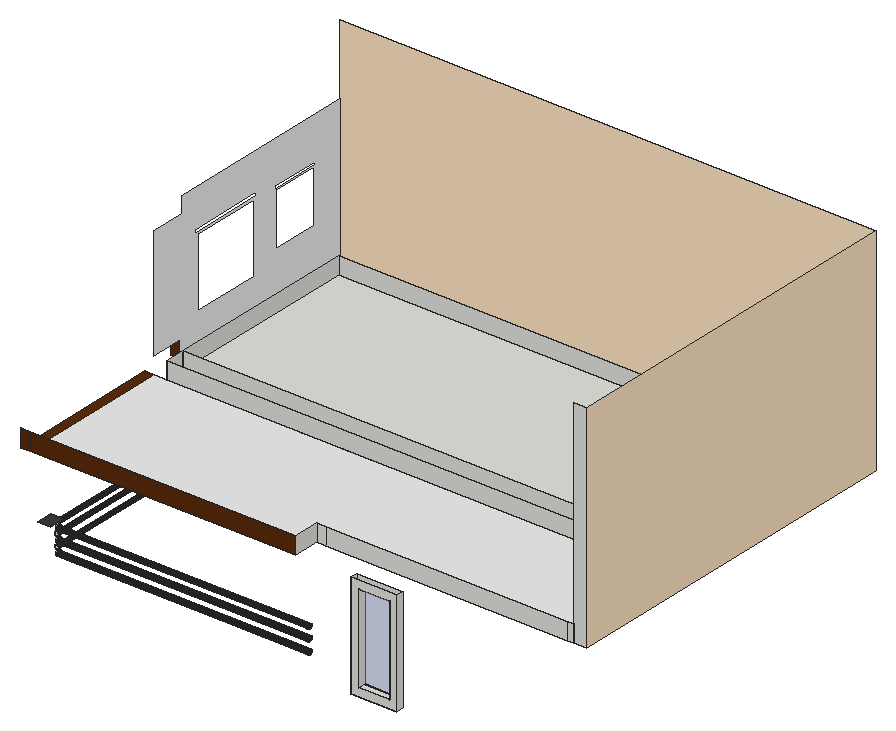
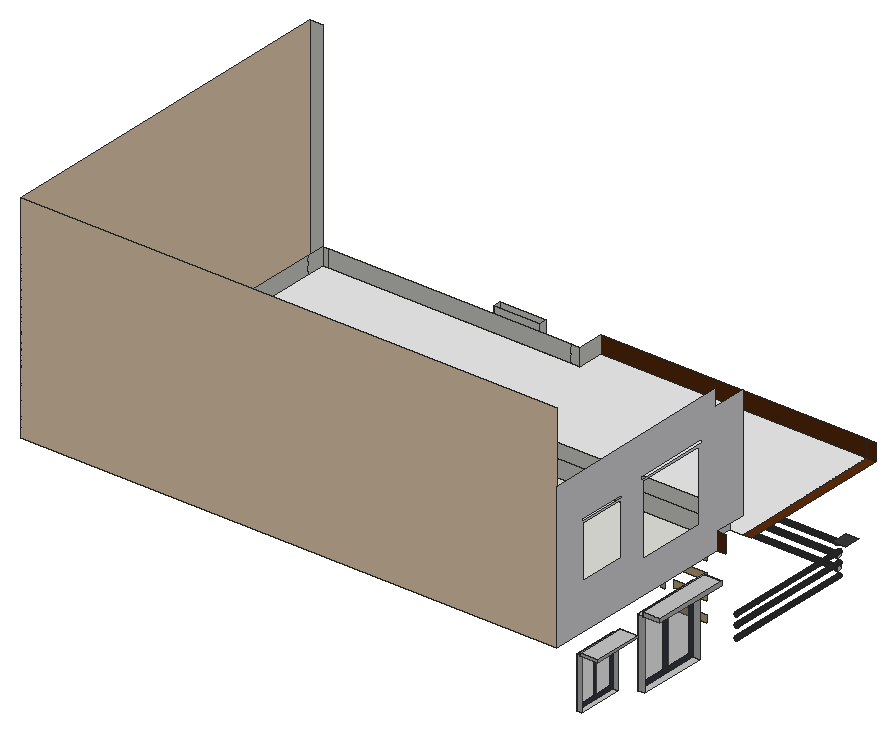
# SketchUp Ruby script. Lengths in inches.
U = 1.inch
M = Sketchup.active_model
def pt(a) = Geom::Point3d.new(a.map { |v| v * U })
def face(e, loops, mat)
  f = e.add_face(loops[0].map { |a| pt(a) })
  loops[1..].each { |l| e.add_face(l.map { |a| pt(a) }).erase! }
  f.material = f.back_material = mat if mat
  f
end
# faces: each face lists its corners as indices into pts; further lists are holes
def faces(e, pts, list, mat = nil) = list.each { |f| face(e, (f[0].is_a?(Array) ? f : [f]).map { |l| l.map { |i| pts[i] } }, mat) }
# xy, xz, yz: faces in a plane at the given z, y or x. An outline is a flat list of corners, or four numbers for a rectangle; further outlines are holes
def ring(l) = l.size == 4 ? [[l[0], l[1]], [l[2], l[1]], [l[2], l[3]], [l[0], l[3]]] : l.each_slice(2).to_a
def flat(e, list, mat, &to3) = list.each { |f| face(e, (f[0].is_a?(Array) ? f : [f]).map { |l| ring(l).map { |u, v| to3.(u, v) } }, mat) }
def xy(e, z, list, mat = nil) = flat(e, list, mat) { |x, y| [x, y, z] }
def xz(e, y, list, mat = nil) = flat(e, list, mat) { |x, z| [x, y, z] }
def yz(e, x, list, mat = nil) = flat(e, list, mat) { |y, z| [x, y, z] }
def lines(e, pts, list) = list.each { |a, b| e.add_line(pt(pts[a]), pt(pts[b])) }
# prism: a flat outline (further loops are holes) pulled along v
def prism(e, loops, v, mat = nil)
  f = face(e, loops, mat); d = Geom::Vector3d.new(v.map { |x| x * U })
  f.pushpull(f.normal.samedirection?(d) ? d.length : -d.length)
end
def box(e, o, s, mat = nil) = prism(e, [[o, [o[0] + s[0], o[1], o[2]], [o[0] + s[0], o[1] + s[1], o[2]], [o[0], o[1] + s[1], o[2]]]], [0, 0, s[2]], mat)
def at(x, y, z, deg = 0) = Geom::Transformation.translation(pt([x, y, z])) * Geom::Transformation.rotation(ORIGIN, Z_AXIS, deg.degrees)
def axes(o, x, y, z) = Geom::Transformation.new([*x, 0, *y, 0, *z, 0, *pt(o).to_a, 1])
def part(name) = M.definitions.add(name)
# library, detail: a bought-in or finely detailed component or shape, given as its bounding box
def library(name, o, s) = part(name).tap { |d| box(d.entities, o, s) }
def detail(e, o, s) = box(e.add_group.entities, o, s)
def put(e, d, t, mat = nil) = e.add_instance(d, t).tap { |i| i.material = mat if mat }
def group(e, t, mat = nil) = e.add_group.tap { |g| g.transformation = t; g.material = mat if mat }.entities
root = M.entities
M.materials.add("[0012_Bisque]").color = [255, 228, 196]
M.materials.add("[0043_SaddleBrown]").color = [91, 44, 12]
M.materials.add("[Blinds Vertical Pattern]").color = [237, 237, 239]
M.materials.add("[Color M02]").color = [198, 198, 198]
M.materials.add("[Color M07]").color = [58, 58, 58]
M.materials.add("[Formica Beige]").color = [211, 187, 149]
M.materials.add("[Formica Laminate Dark]").color = [59, 63, 71]
M.materials.add("[Translucent Glass Gray]").color = [128, 128, 128]
M.materials["[Translucent Glass Gray]"].alpha = 0.5
M.materials.add("[Translucent Glass Safety]").color = [204, 235, 244]
M.materials["[Translucent Glass Safety]"].alpha = 0.5
M.materials.add("[Translucent Glass Sky Reflection]").color = [126, 138, 183]
M.materials["[Translucent Glass Sky Reflection]"].alpha = 0.52
M.materials.add("[Wood Cherry Original]").color = [89, 50, 24]
M.materials.add("[Wood Floor Light]").color = [204, 176, 127]
xy(root,649.8125,[[378.18,386.34,421.12,393.34]])
xy(root,656.84,[[385.21,386.34,414.1,393.34]])
xy(root,659.05,[[73.92,587.21,80.86,651.27]],"[Color M02]")
xy(root,659.52,[[201.38,538.2,275.19,546.63]],"[Formica Beige]")
xy(root,672.3125,[[79.49,512.61,79.89,512.67,80.27,512.82,80.59,513.07,80.84,513.4,81,513.77,81.05,514.18,81,514.58,80.84,514.96,80.59,515.28,80.27,515.53,79.89,515.6875,79.49,515.74,79.08,515.6875,78.7,515.53,78.38,515.28,78.13,514.96,77.98,514.58,77.92,514.18,77.98,513.77,78.13,513.4,78.38,513.07,78.7,512.82,79.08,512.67]])
xy(root,672.79,[[79.49,444.43,79.89,444.48,80.27,444.64,80.59,444.88,80.84,445.21,81,445.59,81.05,445.99,81,446.39,80.84,446.77,80.59,447.09,80.27,447.34,79.89,447.5,79.49,447.55,79.08,447.5,78.7,447.34,78.38,447.09,78.13,446.77,77.98,446.39,77.93,446.02,77.93,445.96,77.98,445.59,78.13,445.21,78.38,444.88,78.7,444.64,79.08,444.48],[77.93,445.96,77.93,446.02,77.92,445.99]])
xy(root,674.0625,[[79.49,476.18,79.89,476.23,80.27,476.39,80.59,476.63,80.84,476.96,81,477.34,81.05,477.74,81,478.14,80.84,478.52,80.59,478.84,80.27,479.09,79.89,479.25,79.49,479.3,79.08,479.25,78.7,479.09,78.38,478.84,78.13,478.52,77.98,478.14,77.92,477.74,77.98,477.34,78.13,476.96,78.38,476.63,78.7,476.39,79.08,476.23]])
xy(root,674.1875,[[268.26,408.99,268.67,409.04,269.04,409.2,269.37,409.45,269.62,409.77,269.77,410.15,269.83,410.55,269.77,410.96,269.62,411.34,269.37,411.66,269.04,411.91,268.67,412.0625,268.26,412.12,267.86,412.0625,267.48,411.91,267.16,411.66,266.91,411.34,266.75,410.96,266.7,410.55,266.75,410.15,266.91,409.77,267.16,409.45,267.48,409.2,267.86,409.04]])
xy(root,674.88,[[204.26,408.99,204.67,409.04,205.04,409.2,205.37,409.45,205.62,409.77,205.77,410.15,205.83,410.55,205.77,410.96,205.62,411.34,205.37,411.66,205.04,411.91,204.67,412.0625,204.26,412.12,203.86,412.0625,203.48,411.91,203.16,411.66,202.91,411.34,202.75,410.96,202.7,410.55,202.75,410.15,202.91,409.77,203.16,409.45,203.48,409.2,203.86,409.04]])
xy(root,675.28,[[73.92,682.92,78.67,724.55]],"[Color M02]")
xy(root,675.42,[[142.95,408.99,143.36,409.04,143.73,409.2,144.06,409.45,144.3,409.77,144.46,410.15,144.51,410.55,144.46,410.96,144.3,411.34,144.06,411.66,143.73,411.91,143.36,412.0625,142.95,412.12,142.55,412.0625,142.17,411.91,141.85,411.66,141.6,411.34,141.44,410.96,141.39,410.55,141.44,410.15,141.6,409.77,141.85,409.45,142.17,409.2,142.55,409.04]])
xy(root,678.5625,[[73.92,403.22,85.98,418.04]],"[Color M07]")
xy(root,722.34,[[73.92,682.92,78.67,724.55]],"[Color M02]")
xy(root,722.4,[[201.38,538.2,275.19,546.63]],"[Formica Beige]")
xy(root,723.11,[[73.92,587.21,80.86,651.27]],"[Color M02]")
xy(root,723.29,[[57.67,680.2,73.92,726.88]],"[Color M02]")
xy(root,724.34,[[57.67,582.96,73.92,654.15]],"[Color M02]")
xy(root,725.66,[[57.67,680.2,73.92,726.88]],"[Color M02]")
xy(root,728.22,[[57.67,582.96,73.92,654.15]],"[Color M02]")
xy(root,739.54,[[385.21,386.34,414.1,393.34]])
xy(root,741.625,[[85.98,538.2,560.26,556.28],[85.98,556.28,560.26,737.09]])
xy(root,741.625,[[65.42,393.34,73.92,538.2]],"[0043_SaddleBrown]")
xy(root,741.625,[[73.92,393.34,73.92,538.2,560.26,538.2,560.26,418.04,320.99,418.04,320.99,393.34]],"[Blinds Vertical Pattern]")
xz(root,386.34,[[[378.18,649.8125,421.12,746.5625],[385.21,656.84,414.1,739.54]]])
xz(root,393.34,[[[378.18,649.8125,421.12,746.5625],[385.21,656.84,414.1,739.54]]])
xz(root,393.34,[[65.42,741.625,73.92,757.5],[73.92,741.625,320.99,757.5]],"[0043_SaddleBrown]")
xz(root,393.34,[[385.21,656.84,414.1,739.54]],"[Translucent Glass Sky Reflection]")
xz(root,418.04,[[79.68,651.2,80.15,651.26,80.58,651.4375,80.96,651.73,81.25,652.1,81.43,652.54,81.49,653.01,81.43,653.48,81.25,653.92,80.96,654.29,80.58,654.58,80.15,654.76,79.68,654.82,79.21,654.76,78.77,654.58,78.4,654.29,78.11,653.92,77.93,653.48,77.87,653.01,77.93,652.54,78.11,652.1,78.4,651.73,78.77,651.4375,79.21,651.26],[79.68,661.95,80.15,662.01,80.58,662.1875,80.96,662.48,81.25,662.85,81.43,663.29,81.49,663.76,81.43,664.23,81.25,664.67,80.96,665.04,80.58,665.33,80.15,665.51,79.68,665.57,79.21,665.51,78.77,665.33,78.4,665.04,78.11,664.67,77.93,664.23,77.87,663.76,77.93,663.29,78.11,662.85,78.4,662.48,78.77,662.1875,79.21,662.01],[79.68,671.45,80.15,671.51,80.58,671.6875,80.96,671.98,81.25,672.35,81.43,672.79,81.49,673.26,81.43,673.73,81.25,674.17,80.96,674.54,80.58,674.83,80.15,675.01,79.68,675.07,79.21,675.01,78.77,674.83,78.4,674.54,78.11,674.17,77.93,673.73,77.87,673.26,77.93,672.79,78.11,672.35,78.4,671.98,78.77,671.6875,79.21,671.51],[320.99,741.625,329.72,757.5],[329.72,741.625,554.62,757.5],
  [554.62,741.625,560.26,757.5],[560.26,741.625,572.32,941.875]])
xz(root,538.2,[[85.98,741.625,560.26,757.5]])
xz(root,538.2,[[106.93,656.78,137.99,663.34],[146.5,671.28,150.06,692.91],[106.93,674.53,137.99,681.09],[106.93,691.28,137.99,697.84],[106.93,707.84,137.99,714.4]],"[Wood Floor Light]")
xz(root,546.63,[[205.69,663.83,220.26,718.09]],"[Translucent Glass Safety]")
xz(root,546.63,[[[201.38,659.52,275.19,722.4],[205.69,663.83,270.89,718.09]],[220.26,663.83,234.83,718.09],[234.83,663.83,241.11,718.09],[241.11,663.83,270.89,718.09]],"[Wood Cherry Original]")
xz(root,556.28,[[85.98,741.625,560.26,757.5]])
xz(root,568.32,[[65.42,741.625,73.92,757.5]],"[0043_SaddleBrown]")
xz(root,582.96,[[57.67,724.34,73.92,728.22]],"[Color M02]")
xz(root,587.21,[[73.92,659.05,80.86,723.11]],"[Color M02]")
xz(root,651.27,[[73.92,659.05,80.86,723.11]],"[Color M02]")
xz(root,654.15,[[57.67,724.34,73.92,728.22]],"[Color M02]")
xz(root,680.2,[[57.67,723.29,73.92,725.66]],"[Color M02]")
xz(root,682.92,[[73.92,675.28,78.67,722.34]],"[Color M02]")
xz(root,724.55,[[73.92,675.28,78.67,722.34]],"[Color M02]")
xz(root,726.88,[[57.67,723.29,73.92,725.66]],"[Color M02]")
xz(root,737.09,[[85.98,741.625,560.26,757.5]])
xz(root,753.91,[[73.92,741.625,572.32,941.875]],"[0012_Bisque]")
yz(root,57.67,[[680.2,723.29,726.88,725.66],[582.96,724.34,654.15,728.22]],"[Color M02]")
yz(root,73.92,[[680.2,723.29,726.88,725.66],[582.96,724.34,654.15,728.22]])
yz(root,73.92,[[[568.32,741.625,568.32,757.5,538.2,757.5,538.2,861.625,569.95,861.625,569.95,876.375,753.91,876.375,753.91,741.625],[589.12,771.97,653.81,836.66],[679.68,784.22,723.8,832.97],[584.97,838.57,656.41,841.76],[678.66,833.97,725.11,836.66]]],"[Blinds Vertical Pattern]")
yz(root,78.67,[[[682.92,675.28,724.55,722.34],[686.33,678.69,721.13,718.93]],[702.23,678.69,705.39,718.93]],"[Formica Laminate Dark]")
yz(root,78.67,[[686.33,678.69,702.23,718.93],[705.39,678.69,721.13,718.93]],"[Translucent Glass Gray]")
yz(root,80.86,[[[587.21,659.05,651.27,723.11],[591.69,663.53,646.79,718.63]],[616.19,663.53,622.25,718.63]],"[Formica Laminate Dark]")
yz(root,80.86,[[591.69,663.53,616.19,718.63],[622.25,663.53,646.79,718.63]],"[Translucent Glass Gray]")
yz(root,85.98,[[410.75,651.38,410.22,651.45,409.72,651.66,409.29,651.99,408.97,652.41,408.76,652.91,408.6875,653.44,408.76,653.98,408.97,654.48,409.29,654.9,409.72,655.23,410.22,655.4375,410.75,655.51,411.29,655.4375,411.78,655.23,412.21,654.9,412.54,654.48,412.74,653.98,412.8125,653.44,412.74,652.91,412.54,652.41,412.21,651.99,411.78,651.66,411.29,651.45],[410.75,662.32,410.22,662.39,409.72,662.6,409.29,662.92,408.97,663.35,408.76,663.85,408.6875,664.38,408.76,664.92,408.97,665.41,409.29,665.84,409.72,666.17,410.22,666.375,410.75,666.44,411.29,666.375,411.78,666.17,412.21,665.84,412.54,665.41,412.74,664.92,412.8125,664.38,412.74,663.85,412.54,663.35,412.21,662.92,411.78,662.6,411.29,662.39],[410.75,672.82,410.22,672.89,409.72,673.1,409.29,673.42,408.97,673.85,408.76,674.35,408.6875,674.88,408.76,675.42,408.97,675.91,409.29,676.34,409.72,676.67,410.22,676.875,410.75,676.94,411.29,676.875,411.78,676.67,412.21,676.34,412.54,675.91,412.74,675.42,412.8125,674.88,412.74,674.35,412.54,673.85,412.21,673.42,411.78,673.1,411.29,672.89],[538.2,741.625,556.28,757.5],[556.28,741.625,737.09,757.5]])
yz(root,201.38,[[538.2,659.52,546.63,722.4]],"[Formica Beige]")
yz(root,275.19,[[538.2,659.52,546.63,722.4]],"[Formica Beige]")
yz(root,320.99,[[393.34,741.625,418.04,757.5]])
yz(root,378.18,[[386.34,649.8125,393.34,746.5625]])
yz(root,385.21,[[386.34,656.84,393.34,739.54]])
yz(root,414.1,[[386.34,656.84,393.34,739.54]])
yz(root,421.12,[[386.34,649.8125,393.34,746.5625]])
yz(root,560.26,[[418.04,741.625,434.85,757.5],[434.85,741.625,538.2,757.5],[538.2,741.625,556.28,757.5],[556.28,741.625,737.09,757.5]])
yz(root,572.32,[[418.04,741.625,753.91,941.875]],"[0012_Bisque]")
p = [[79.68,418.04,651.2],[79.21,418.04,651.26],[79.21,538.2,651.26],[79.68,538.2,651.2],[80.15,418.04,651.26],[80.15,538.2,651.26],
  [78.77,418.04,651.4375],[78.77,538.2,651.4375],[80.58,418.04,651.4375],[80.58,538.2,651.4375],[85.98,410.22,651.45],[85.98,410.75,651.38],
  [320.99,410.75,651.38],[320.99,410.22,651.45],[85.98,411.29,651.45],[320.99,411.29,651.45],[78.4,418.04,651.73],[78.4,538.2,651.73],
  [80.96,418.04,651.73],[80.96,538.2,651.73],[85.98,409.72,651.66],[320.99,409.72,651.66],[85.98,411.78,651.66],[320.99,411.78,651.66],
  [85.98,409.29,651.99],[320.99,409.29,651.99],[85.98,412.21,651.99],[320.99,412.21,651.99],[78.11,418.04,652.1],[78.11,538.2,652.1],
  [81.25,418.04,652.1],[81.25,538.2,652.1],[85.98,408.97,652.41],[320.99,408.97,652.41],[85.98,412.54,652.41],[320.99,412.54,652.41],
  [77.93,418.04,652.54],[77.93,538.2,652.54],[81.43,418.04,652.54],[81.43,538.2,652.54],[85.98,408.76,652.91],[320.99,408.76,652.91],
  [85.98,412.74,652.91],[320.99,412.74,652.91],[77.87,418.04,653.01],[77.87,538.2,653.01],[81.49,418.04,653.01],[81.49,538.2,653.01],
  [85.98,408.6875,653.44],[320.99,408.6875,653.44],[85.98,412.8125,653.44],[320.99,412.8125,653.44],[77.93,418.04,653.48],[77.93,538.2,653.48],
  [81.43,418.04,653.48],[81.43,538.2,653.48],[85.98,408.76,653.98],[320.99,408.76,653.98],[85.98,412.74,653.98],[320.99,412.74,653.98],
  [78.11,418.04,653.92],[78.11,538.2,653.92],[81.25,418.04,653.92],[81.25,538.2,653.92],[78.4,418.04,654.29],[78.4,538.2,654.29],
  [80.96,418.04,654.29],[80.96,538.2,654.29],[85.98,408.97,654.48],[320.99,408.97,654.48],[85.98,412.54,654.48],[320.99,412.54,654.48],
  [78.77,418.04,654.58],[78.77,538.2,654.58],[80.58,418.04,654.58],[80.58,538.2,654.58],[85.98,409.29,654.9],[320.99,409.29,654.9],
  [85.98,412.21,654.9],[320.99,412.21,654.9],[79.21,418.04,654.76],[79.21,538.2,654.76],[80.15,418.04,654.76],[80.15,538.2,654.76],
  [79.68,418.04,654.82],[79.68,538.2,654.82],[85.98,409.72,655.23],[320.99,409.72,655.23],[85.98,411.78,655.23],[320.99,411.78,655.23],
  [85.98,410.22,655.4375],[320.99,410.22,655.4375],[85.98,411.29,655.4375],[320.99,411.29,655.4375],[85.98,410.75,655.51],[320.99,410.75,655.51],
  [79.68,418.04,661.95],[79.21,418.04,662.01],[79.21,538.2,662.01],[79.68,538.2,661.95],[80.15,418.04,662.01],[80.15,538.2,662.01],
  [78.77,418.04,662.1875],[78.77,538.2,662.1875],[80.58,418.04,662.1875],[80.58,538.2,662.1875],[78.4,418.04,662.48],[78.4,538.2,662.48],
  [80.96,418.04,662.48],[80.96,538.2,662.48],[85.98,410.22,662.39],[85.98,410.75,662.32],[320.99,410.75,662.32],[320.99,410.22,662.39],
  [85.98,411.29,662.39],[320.99,411.29,662.39],[85.98,409.72,662.6],[320.99,409.72,662.6],[85.98,411.78,662.6],[320.99,411.78,662.6],
  [78.11,418.04,662.85],[78.11,538.2,662.85],[81.25,418.04,662.85],[81.25,538.2,662.85],[85.98,409.29,662.92],[320.99,409.29,662.92],
  [85.98,412.21,662.92],[320.99,412.21,662.92],[85.98,408.97,663.35],[320.99,408.97,663.35],[85.98,412.54,663.35],[320.99,412.54,663.35],
  [77.93,418.04,663.29],[77.93,538.2,663.29],[81.43,418.04,663.29],[81.43,538.2,663.29],[77.87,418.04,663.76],[77.87,538.2,663.76],
  [81.49,418.04,663.76],[81.49,538.2,663.76],[85.98,408.76,663.85],[320.99,408.76,663.85],[85.98,412.74,663.85],[320.99,412.74,663.85],
  [85.98,408.6875,664.38],[320.99,408.6875,664.38],[85.98,412.8125,664.38],[320.99,412.8125,664.38],[77.93,418.04,664.23],[77.93,538.2,664.23],
  [81.43,418.04,664.23],[81.43,538.2,664.23],[78.11,418.04,664.67],[78.11,538.2,664.67],[81.25,418.04,664.67],[81.25,538.2,664.67],
  [85.98,408.76,664.92],[320.99,408.76,664.92],[85.98,412.74,664.92],[320.99,412.74,664.92],[78.4,418.04,665.04],[78.4,538.2,665.04],
  [80.96,418.04,665.04],[80.96,538.2,665.04],[85.98,408.97,665.41],[320.99,408.97,665.41],[85.98,412.54,665.41],[320.99,412.54,665.41],
  [78.77,418.04,665.33],[78.77,538.2,665.33],[80.58,418.04,665.33],[80.58,538.2,665.33],[79.21,418.04,665.51],[79.21,538.2,665.51],
  [80.15,418.04,665.51],[80.15,538.2,665.51],[85.98,409.29,665.84],[320.99,409.29,665.84],[85.98,412.21,665.84],[320.99,412.21,665.84],
  [79.68,418.04,665.57],[79.68,538.2,665.57],[85.98,409.72,666.17],[320.99,409.72,666.17],[85.98,411.78,666.17],[320.99,411.78,666.17],
  [85.98,410.22,666.375],[320.99,410.22,666.375],[85.98,411.29,666.375],[320.99,411.29,666.375],[85.98,410.75,666.44],[320.99,410.75,666.44],
  [79.68,418.04,671.45],[79.21,418.04,671.51],[79.21,538.2,671.51],[79.68,538.2,671.45],[80.15,418.04,671.51],[80.15,538.2,671.51],
  [78.77,418.04,671.6875],[78.77,538.2,671.6875],[80.58,418.04,671.6875],[80.58,538.2,671.6875],[78.4,418.04,671.98],[78.4,538.2,671.98],
  [80.96,418.04,671.98],[80.96,538.2,671.98],[78.11,418.04,672.35],[78.11,538.2,672.35],[81.25,418.04,672.35],[81.25,538.2,672.35],
  [77.93,418.04,672.79],[77.93,445.96,672.79],[77.93,446.02,672.79],[77.93,538.2,672.79],[81.43,418.04,672.79],[81.43,538.2,672.79],
  [85.98,410.22,672.89],[85.98,410.75,672.82],[320.99,410.75,672.82],[320.99,410.22,672.89],[85.98,411.29,672.89],[320.99,411.29,672.89],
  [77.87,418.04,673.26],[77.87,538.2,673.26],[81.49,418.04,673.26],[81.49,538.2,673.26],[85.98,409.72,673.1],[320.99,409.72,673.1],
  [85.98,411.78,673.1],[320.99,411.78,673.1],[85.98,409.29,673.42],[320.99,409.29,673.42],[85.98,412.21,673.42],[320.99,412.21,673.42],
  [77.93,418.04,673.73],[77.93,538.2,673.73],[81.43,418.04,673.73],[81.43,538.2,673.73],[85.98,408.97,673.85],[320.99,408.97,673.85],
  [85.98,412.54,673.85],[320.99,412.54,673.85],[78.11,418.04,674.17],[78.11,538.2,674.17],[81.25,418.04,674.17],[81.25,538.2,674.17],
  [85.98,408.76,674.35],[320.99,408.76,674.35],[85.98,412.74,674.35],[320.99,412.74,674.35],[78.4,418.04,674.54],[78.4,538.2,674.54],
  [80.96,418.04,674.54],[80.96,538.2,674.54],[85.98,408.6875,674.88],[320.99,408.6875,674.88],[85.98,412.8125,674.88],[320.99,412.8125,674.88],
  [78.77,418.04,674.83],[78.77,538.2,674.83],[80.58,418.04,674.83],[80.58,538.2,674.83],[79.21,418.04,675.01],[79.21,538.2,675.01],
  [80.15,418.04,675.01],[80.15,538.2,675.01],[85.98,408.76,675.42],[320.99,408.76,675.42],[85.98,412.74,675.42],[320.99,412.74,675.42],
  [79.68,418.04,675.07],[79.68,538.2,675.07],[85.98,408.97,675.91],[320.99,408.97,675.91],[85.98,412.54,675.91],[320.99,412.54,675.91],
  [85.98,409.29,676.34],[320.99,409.29,676.34],[85.98,412.21,676.34],[320.99,412.21,676.34],[85.98,409.72,676.67],[320.99,409.72,676.67],
  [85.98,411.78,676.67],[320.99,411.78,676.67],[85.98,410.22,676.875],[320.99,410.22,676.875],[85.98,411.29,676.875],[320.99,411.29,676.875],
  [85.98,410.75,676.94],[320.99,410.75,676.94]]
faces(root,p,[[0,1,2,3],[4,0,3,5],[1,6,7,2],[8,4,5,9],[10,11,12,13],[11,14,15,12],[6,16,17,7],[18,8,9,19],
  [20,10,13,21],[14,22,23,15],[24,20,21,25],[22,26,27,23],[16,28,29,17],[30,18,19,31],[32,24,25,33],[26,34,35,27],
  [28,36,37,29],[38,30,31,39],[40,32,33,41],[34,42,43,35],[36,44,45,37],[46,38,39,47],[48,40,41,49],[42,50,51,43],
  [44,52,53,45],[54,46,47,55],[56,48,49,57],[50,58,59,51],[52,60,61,53],[62,54,55,63],[60,64,65,61],[66,62,63,67],
  [68,56,57,69],[58,70,71,59],[64,72,73,65],[74,66,67,75],[76,68,69,77],[70,78,79,71],[72,80,81,73],[82,74,75,83],
  [80,84,85,81],[84,82,83,85],[86,76,77,87],[78,88,89,79],[90,86,87,91],[88,92,93,89],[94,90,91,95],[92,94,95,93],
  [96,97,98,99],[100,96,99,101],[97,102,103,98],[104,100,101,105],[102,106,107,103],[108,104,105,109],[110,111,112,113],[111,114,115,112],
  [116,110,113,117],[114,118,119,115],[106,120,121,107],[122,108,109,123],[124,116,117,125],[118,126,127,119],[128,124,125,129],[126,130,131,127],
  [120,132,133,121],[134,122,123,135],[132,136,137,133],[138,134,135,139],[140,128,129,141],[130,142,143,131],[144,140,141,145],[142,146,147,143],
  [136,148,149,137],[150,138,139,151],[148,152,153,149],[154,150,151,155],[156,144,145,157],[146,158,159,147],[152,160,161,153],[162,154,155,163],
  [164,156,157,165],[158,166,167,159],[160,168,169,161],[170,162,163,171],[168,172,173,169],[174,170,171,175],[176,164,165,177],[166,178,179,167],
  [172,180,181,173],[180,174,175,181],[182,176,177,183],[178,184,185,179],[186,182,183,187],[184,188,189,185],[190,186,187,191],[188,190,191,189],
  [192,193,194,195],[196,192,195,197],[193,198,199,194],[200,196,197,201],[198,202,203,199],[204,200,201,205],[202,206,207,203],[208,204,205,209],
  [206,210,211,212,213,207],[214,208,209,215],[216,217,218,219],[217,220,221,218],[210,222,223,213,212,211],[224,214,215,225],[226,216,219,227],[220,228,229,221],
  [230,226,227,231],[228,232,233,229],[222,234,235,223],[236,224,225,237],[238,230,231,239],[232,240,241,233],[234,242,243,235],[244,236,237,245],
  [246,238,239,247],[240,248,249,241],[242,250,251,243],[252,244,245,253],[254,246,247,255],[248,256,257,249],[250,258,259,251],[260,252,253,261],
  [258,262,263,259],[264,260,261,265],[266,254,255,267],[256,268,269,257],[262,270,271,263],[270,264,265,271],[272,266,267,273],[268,274,275,269],
  [276,272,273,277],[274,278,279,275],[280,276,277,281],[278,282,283,279],[284,280,281,285],[282,286,287,283],[288,284,285,289],[286,288,289,287]],"[Color M07]")
